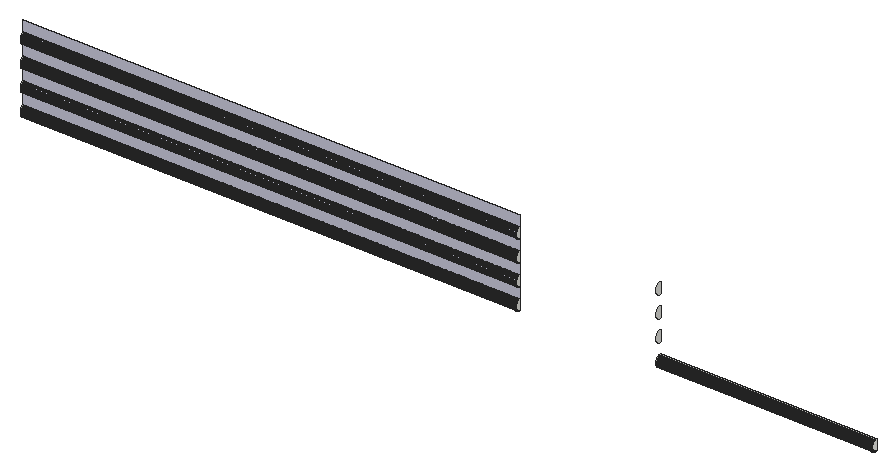
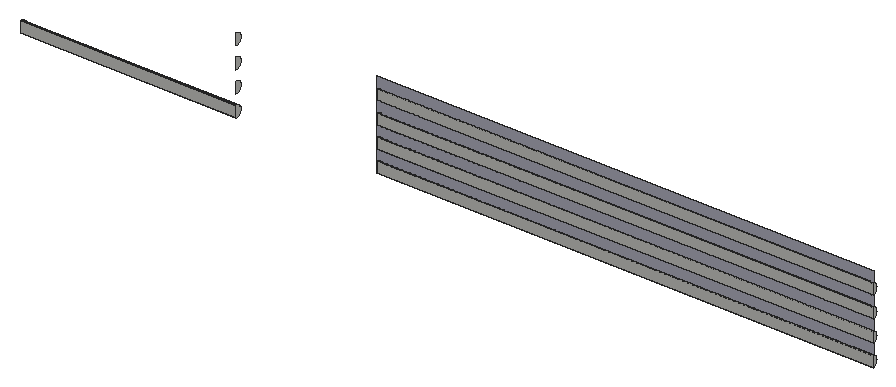
# SketchUp Ruby script. Lengths in millimetres.
U = 1.mm
M = Sketchup.active_model
def pt(a) = Geom::Point3d.new(a.map { |v| v * U })
def face(e, loops, mat)
  f = e.add_face(loops[0].map { |a| pt(a) })
  loops[1..].each { |l| e.add_face(l.map { |a| pt(a) }).erase! }
  f.material = f.back_material = mat if mat
  f
end
# faces: each face lists its corners as indices into pts; further lists are holes
def faces(e, pts, list, mat = nil) = list.each { |f| face(e, (f[0].is_a?(Array) ? f : [f]).map { |l| l.map { |i| pts[i] } }, mat) }
# xy, xz, yz: faces in a plane at the given z, y or x. An outline is a flat list of corners, or four numbers for a rectangle; further outlines are holes
def ring(l) = l.size == 4 ? [[l[0], l[1]], [l[2], l[1]], [l[2], l[3]], [l[0], l[3]]] : l.each_slice(2).to_a
def flat(e, list, mat, &to3) = list.each { |f| face(e, (f[0].is_a?(Array) ? f : [f]).map { |l| ring(l).map { |u, v| to3.(u, v) } }, mat) }
def xy(e, z, list, mat = nil) = flat(e, list, mat) { |x, y| [x, y, z] }
def xz(e, y, list, mat = nil) = flat(e, list, mat) { |x, z| [x, y, z] }
def yz(e, x, list, mat = nil) = flat(e, list, mat) { |y, z| [x, y, z] }
def lines(e, pts, list) = list.each { |a, b| e.add_line(pt(pts[a]), pt(pts[b])) }
# prism: a flat outline (further loops are holes) pulled along v
def prism(e, loops, v, mat = nil)
  f = face(e, loops, mat); d = Geom::Vector3d.new(v.map { |x| x * U })
  f.pushpull(f.normal.samedirection?(d) ? d.length : -d.length)
end
def box(e, o, s, mat = nil) = prism(e, [[o, [o[0] + s[0], o[1], o[2]], [o[0] + s[0], o[1] + s[1], o[2]], [o[0], o[1] + s[1], o[2]]]], [0, 0, s[2]], mat)
def at(x, y, z, deg = 0) = Geom::Transformation.translation(pt([x, y, z])) * Geom::Transformation.rotation(ORIGIN, Z_AXIS, deg.degrees)
def axes(o, x, y, z) = Geom::Transformation.new([*x, 0, *y, 0, *z, 0, *pt(o).to_a, 1])
def part(name) = M.definitions.add(name)
# library, detail: a bought-in or finely detailed component or shape, given as its bounding box
def library(name, o, s) = part(name).tap { |d| box(d.entities, o, s) }
def detail(e, o, s) = box(e.add_group.entities, o, s)
def put(e, d, t, mat = nil) = e.add_instance(d, t).tap { |i| i.material = mat if mat }
def group(e, t, mat = nil) = e.add_group.tap { |g| g.transformation = t; g.material = mat if mat }.entities
root = M.entities
M.materials.add("[0116_Lavender]").color = [197, 197, 214]
xz(root,16548.1,[[11038.5,8702.7,25059.3,9007.5],[29021.7,8702.7,35117.7,9007.5],[11038.5,9312.3,25059.3,9617.1],[11038.5,9921.9,25059.3,10226.7],[11038.5,10531.5,25059.3,10836.3]])
xz(root,16548.1,[[11038.5,9007.5,25059.3,9312.3],[11038.5,9617.1,25059.3,9921.9],[11038.5,10226.7,25059.3,10531.5],[11038.5,10836.3,25059.3,11141.1]],"[0116_Lavender]")
yz(root,11038.5,[[16548.1,8702.7,16536.2,8708,16524.8,8714.3,16514,8721.4,16503.7,8729.4,16494.1,8738.2,16485.2,8747.7,16477.1,8757.8,16469.8,8768.6,16463.4,8779.9,16458,8791.7,16453.4,8803.9,16449.9,8816.4,16447.3,8829.2,16445.8,8842.1,16445.3,8855.1,16445.8,8868.1,16447.3,8881,16449.9,8893.7,16453.4,8906.2,16458,8918.4,16463.4,8930.2,16469.8,8941.5,16477.1,8952.3,16485.2,8962.5,16494.1,8972,16503.7,8980.8,16514,8988.7,16524.8,8995.9,16536.2,9002.1,16548.1,9007.5],[16548.1,9312.3,16536.2,9317.6,16524.8,9323.9,16514,9331,16503.7,9339,16494.1,9347.8,16485.2,9357.3,16477.1,9367.4,16469.8,9378.2,16463.4,9389.5,16458,9401.3,16453.4,9413.5,16449.9,9426,16447.3,9438.8,16445.8,9451.7,16445.3,9464.7,16445.8,9477.7,16447.3,9490.6,16449.9,9503.3,16453.4,9515.8,16458,9528,16463.4,9539.8,16469.8,9551.1,16477.1,9561.9,16485.2,9572.1,16494.1,9581.6,16503.7,9590.4,16514,9598.3,16524.8,9605.5,16536.2,9611.7,16548.1,9617.1],[16548.1,9921.9,16536.2,9927.2,16524.8,9933.5,16514,9940.6,16503.7,9948.6,16494.1,9957.4,16485.2,9966.9,16477.1,9977,16469.8,9987.8,16463.4,9999.1,16458,10010.9,16453.4,10023.1,16449.9,10035.6,16447.3,10048.4,16445.8,10061.3,16445.3,10074.3,16445.8,10087.3,16447.3,10100.2,16449.9,10112.9,16453.4,10125.4,16458,10137.6,16463.4,10149.4,16469.8,10160.7,16477.1,10171.5,16485.2,10181.7,16494.1,10191.2,16503.7,10200,16514,10207.9,16524.8,10215.1,16536.2,10221.3,16548.1,10226.7],[16548.1,10531.5,16536.2,10536.8,16524.8,10543.1,16514,10550.2,16503.7,10558.2,16494.1,10567,16485.2,10576.5,16477.1,10586.6,16469.8,10597.4,16463.4,10608.7,16458,10620.5,16453.4,10632.7,16449.9,10645.2,16447.3,10658,16445.8,10670.9,16445.3,10683.9,16445.8,10696.9,16447.3,10709.8,16449.9,10722.5,16453.4,10735,16458,10747.2,16463.4,10759,16469.8,10770.3,16477.1,10781.1,16485.2,10791.3,16494.1,10800.8,16503.7,10809.6,16514,10817.5,16524.8,10824.7,16536.2,10830.9,16548.1,10836.3]])
yz(root,25059.3,[[16548.1,8702.7,16548.1,9007.5,16536.2,9002.1,16524.8,8995.9,16514,8988.7,16503.7,8980.8,16494.1,8972,16485.2,8962.5,16477.1,8952.3,16469.8,8941.5,16463.4,8930.2,16458,8918.4,16453.4,8906.2,16449.9,8893.7,16447.3,8881,16445.8,8868.1,16445.3,8855.1,16445.8,8842.1,16447.3,8829.2,16449.9,8816.4,16453.4,8803.9,16458,8791.7,16463.4,8779.9,16469.8,8768.6,16477.1,8757.8,16485.2,8747.7,16494.1,8738.2,16503.7,8729.4,16514,8721.4,16524.8,8714.3,16536.2,8708],[16548.1,9312.3,16548.1,9617.1,16536.2,9611.7,16524.8,9605.5,16514,9598.3,16503.7,9590.4,16494.1,9581.6,16485.2,9572.1,16477.1,9561.9,16469.8,9551.1,16463.4,9539.8,16458,9528,16453.4,9515.8,16449.9,9503.3,16447.3,9490.6,16445.8,9477.7,16445.3,9464.7,16445.8,9451.7,16447.3,9438.8,16449.9,9426,16453.4,9413.5,16458,9401.3,16463.4,9389.5,16469.8,9378.2,16477.1,9367.4,16485.2,9357.3,16494.1,9347.8,16503.7,9339,16514,9331,16524.8,9323.9,16536.2,9317.6],[16548.1,9921.9,16548.1,10226.7,16536.2,10221.3,16524.8,10215.1,16514,10207.9,16503.7,10200,16494.1,10191.2,16485.2,10181.7,16477.1,10171.5,16469.8,10160.7,16463.4,10149.4,16458,10137.6,16453.4,10125.4,16449.9,10112.9,16447.3,10100.2,16445.8,10087.3,16445.3,10074.3,16445.8,10061.3,16447.3,10048.4,16449.9,10035.6,16453.4,10023.1,16458,10010.9,16463.4,9999.1,16469.8,9987.8,16477.1,9977,16485.2,9966.9,16494.1,9957.4,16503.7,9948.6,16514,9940.6,16524.8,9933.5,16536.2,9927.2],[16548.1,10531.5,16548.1,10836.3,16536.2,10830.9,16524.8,10824.7,16514,10817.5,16503.7,10809.6,16494.1,10800.8,16485.2,10791.3,16477.1,10781.1,16469.8,10770.3,16463.4,10759,16458,10747.2,16453.4,10735,16449.9,10722.5,16447.3,10709.8,16445.8,10696.9,16445.3,10683.9,16445.8,10670.9,16447.3,10658,16449.9,10645.2,16453.4,10632.7,16458,10620.5,16463.4,10608.7,16469.8,10597.4,16477.1,10586.6,16485.2,10576.5,16494.1,10567,16503.7,10558.2,16514,10550.2,16524.8,10543.1,16536.2,10536.8]])
yz(root,29021.7,[[16548.1,8702.7,16540.1,8702.9,16532.2,8703.5,16524.3,8704.6,16516.4,8706,16508.7,8707.9,16501,8710.1,16493.5,8712.8,16486.1,8715.9,16478.9,8719.3,16471.9,8723.1,16465.1,8727.3,16458.5,8731.8,16452.2,8736.6,16446.1,8741.8,16440.3,8747.3,16434.8,8753.1,16429.7,8759.2,16424.8,8765.5,16420.3,8772.1,16416.1,8778.9,16412.3,8785.9,16408.9,8793.1,16405.8,8800.5,16403.2,8808,16400.9,8815.6,16399,8823.4,16397.6,8831.2,16396.5,8839.1,16395.9,8847.1,16395.7,8855.1,16395.9,8863.1,16396.5,8871,16397.6,8878.9,16399,8886.8,16400.9,8894.5,16403.2,8902.2,16405.8,8909.7,16408.9,8917.1,16412.3,8924.3,16416.1,8931.3,16420.3,8938.1,16424.8,8944.7,16429.7,8951,16434.8,8957.1,16440.3,8962.8,16446.1,8968.3,16452.2,8973.5,16458.5,8978.4,16465.1,8982.9,16471.9,8987.1,16478.9,8990.9,16486.1,8994.3,16493.5,8997.4,16501,9000,16508.7,9002.3,16516.4,9004.1,16524.3,9005.6,16532.2,9006.6,16540.1,9007.3,16548.1,9007.5],[16548.1,9312.3,16540.1,9312.5,16532.2,9313.1,16524.3,9314.2,16516.4,9315.6,16508.7,9317.5,16501,9319.7,16493.5,9322.4,16486.1,9325.5,16478.9,9328.9,16471.9,9332.7,16465.1,9336.9,16458.5,9341.4,16452.2,9346.2,16446.1,9351.4,16440.3,9356.9,16434.8,9362.7,16429.7,9368.8,16424.8,9375.1,16420.3,9381.7,16416.1,9388.5,16412.3,9395.5,16408.9,9402.7,16405.8,9410.1,16403.2,9417.6,16400.9,9425.2,16399,9433,16397.6,9440.8,16396.5,9448.7,16395.9,9456.7,16395.7,9464.7,16395.9,9472.7,16396.5,9480.6,16397.6,9488.5,16399,9496.4,16400.9,9504.1,16403.2,9511.8,16405.8,9519.3,16408.9,9526.7,16412.3,9533.9,16416.1,9540.9,16420.3,9547.7,16424.8,9554.3,16429.7,9560.6,16434.8,9566.7,16440.3,9572.4,16446.1,9577.9,16452.2,9583.1,16458.5,9588,16465.1,9592.5,16471.9,9596.7,16478.9,9600.5,16486.1,9603.9,16493.5,9607,16501,9609.6,16508.7,9611.9,16516.4,9613.7,16524.3,9615.2,16532.2,9616.2,16540.1,9616.9,16548.1,9617.1],[16548.1,9921.9,16540.1,9922.1,16532.2,9922.7,16524.3,9923.8,16516.4,9925.2,16508.7,9927.1,16501,9929.3,16493.5,9932,16486.1,9935.1,16478.9,9938.5,16471.9,9942.3,16465.1,9946.5,16458.5,9951,16452.2,9955.8,16446.1,9961,16440.3,9966.5,16434.8,9972.3,16429.7,9978.4,16424.8,9984.7,16420.3,9991.3,16416.1,9998.1,16412.3,10005.1,16408.9,10012.3,16405.8,10019.7,16403.2,10027.2,16400.9,10034.8,16399,10042.6,16397.6,10050.4,16396.5,10058.3,16395.9,10066.3,16395.7,10074.3,16395.9,10082.3,16396.5,10090.2,16397.6,10098.1,16399,10106,16400.9,10113.7,16403.2,10121.4,16405.8,10128.9,16408.9,10136.3,16412.3,10143.5,16416.1,10150.5,16420.3,10157.3,16424.8,10163.9,16429.7,10170.2,16434.8,10176.3,16440.3,10182,16446.1,10187.5,16452.2,10192.7,16458.5,10197.6,16465.1,10202.1,16471.9,10206.3,16478.9,10210.1,16486.1,10213.5,16493.5,10216.6,16501,10219.2,16508.7,10221.5,16516.4,10223.3,16524.3,10224.8,16532.2,10225.8,16540.1,10226.5,16548.1,10226.7],[16548.1,10531.5,16540.1,10531.7,16532.2,10532.3,16524.3,10533.4,16516.4,10534.8,16508.7,10536.7,16501,10538.9,16493.5,10541.6,16486.1,10544.7,16478.9,10548.1,16471.9,10551.9,16465.1,10556.1,16458.5,10560.6,16452.2,10565.4,16446.1,10570.6,16440.3,10576.1,16434.8,10581.9,16429.7,10588,16424.8,10594.3,16420.3,10600.9,16416.1,10607.7,16412.3,10614.7,16408.9,10621.9,16405.8,10629.3,16403.2,10636.8,16400.9,10644.4,16399,10652.2,16397.6,10660,16396.5,10667.9,16395.9,10675.9,16395.7,10683.9,16395.9,10691.9,16396.5,10699.8,16397.6,10707.7,16399,10715.6,16400.9,10723.3,16403.2,10731,16405.8,10738.5,16408.9,10745.9,16412.3,10753.1,16416.1,10760.1,16420.3,10766.9,16424.8,10773.5,16429.7,10779.8,16434.8,10785.9,16440.3,10791.6,16446.1,10797.1,16452.2,10802.3,16458.5,10807.2,16465.1,10811.7,16471.9,10815.9,16478.9,10819.7,16486.1,10823.1,16493.5,10826.2,16501,10828.8,16508.7,10831.1,16516.4,10832.9,16524.3,10834.4,16532.2,10835.4,16540.1,10836.1,16548.1,10836.3]])
p = [[25059.3,16548.1,8702.7],[25059.3,16536.2,8708],[11038.5,16536.2,8708],[11038.5,16548.1,8702.7],[35117.7,16548.1,8702.7],[35117.7,16540.1,8702.9],
  [29021.7,16540.1,8702.9],[29021.7,16548.1,8702.7],[35117.7,16532.2,8703.5],[29021.7,16532.2,8703.5],[35117.7,16524.3,8704.6],[29021.7,16524.3,8704.6],
  [35117.7,16516.4,8706],[29021.7,16516.4,8706],[35117.7,16508.7,8707.9],[29021.7,16508.7,8707.9],[35117.7,16501,8710.1],[29021.7,16501,8710.1],
  [25059.3,16524.8,8714.3],[11038.5,16524.8,8714.3],[35117.7,16493.5,8712.8],[29021.7,16493.5,8712.8],[35117.7,16486.1,8715.9],[29021.7,16486.1,8715.9],
  [25059.3,16514,8721.4],[11038.5,16514,8721.4],[35117.7,16478.9,8719.3],[29021.7,16478.9,8719.3],[35117.7,16471.9,8723.1],[29021.7,16471.9,8723.1],
  [25059.3,16503.7,8729.4],[11038.5,16503.7,8729.4],[35117.7,16465.1,8727.3],[29021.7,16465.1,8727.3],[35117.7,16458.5,8731.8],[29021.7,16458.5,8731.8],
  [25059.3,16494.1,8738.2],[11038.5,16494.1,8738.2],[35117.7,16452.2,8736.6],[29021.7,16452.2,8736.6],[35117.7,16446.1,8741.8],[29021.7,16446.1,8741.8],
  [25059.3,16485.2,8747.7],[11038.5,16485.2,8747.7],[35117.7,16440.3,8747.3],[29021.7,16440.3,8747.3],[35117.7,16434.8,8753.1],[29021.7,16434.8,8753.1],
  [25059.3,16477.1,8757.8],[11038.5,16477.1,8757.8],[35117.7,16429.7,8759.2],[29021.7,16429.7,8759.2],[25059.3,16469.8,8768.6],[11038.5,16469.8,8768.6],
  [35117.7,16424.8,8765.5],[29021.7,16424.8,8765.5],[35117.7,16420.3,8772.1],[29021.7,16420.3,8772.1],[25059.3,16463.4,8779.9],[11038.5,16463.4,8779.9],
  [35117.7,16416.1,8778.9],[29021.7,16416.1,8778.9],[35117.7,16412.3,8785.9],[29021.7,16412.3,8785.9],[25059.3,16458,8791.7],[11038.5,16458,8791.7],
  [35117.7,16408.9,8793.1],[29021.7,16408.9,8793.1],[25059.3,16453.4,8803.9],[11038.5,16453.4,8803.9],[35117.7,16405.8,8800.5],[29021.7,16405.8,8800.5],
  [35117.7,16403.2,8808],[29021.7,16403.2,8808],[25059.3,16449.9,8816.4],[11038.5,16449.9,8816.4],[35117.7,16400.9,8815.6],[29021.7,16400.9,8815.6],
  [35117.7,16399,8823.4],[29021.7,16399,8823.4],[25059.3,16447.3,8829.2],[11038.5,16447.3,8829.2],[35117.7,16397.6,8831.2],[29021.7,16397.6,8831.2],
  [25059.3,16445.8,8842.1],[11038.5,16445.8,8842.1],[35117.7,16396.5,8839.1],[29021.7,16396.5,8839.1],[35117.7,16395.9,8847.1],[29021.7,16395.9,8847.1],
  [25059.3,16445.3,8855.1],[11038.5,16445.3,8855.1],[35117.7,16395.7,8855.1],[29021.7,16395.7,8855.1],[35117.7,16395.9,8863.1],[29021.7,16395.9,8863.1],
  [25059.3,16445.8,8868.1],[11038.5,16445.8,8868.1],[35117.7,16396.5,8871],[29021.7,16396.5,8871],[25059.3,16447.3,8881],[11038.5,16447.3,8881],
  [35117.7,16397.6,8878.9],[29021.7,16397.6,8878.9],[35117.7,16399,8886.8],[29021.7,16399,8886.8],[25059.3,16449.9,8893.7],[11038.5,16449.9,8893.7],
  [35117.7,16400.9,8894.5],[29021.7,16400.9,8894.5],[25059.3,16453.4,8906.2],[11038.5,16453.4,8906.2],[35117.7,16403.2,8902.2],[29021.7,16403.2,8902.2],
  [35117.7,16405.8,8909.7],[29021.7,16405.8,8909.7],[25059.3,16458,8918.4],[11038.5,16458,8918.4],[35117.7,16408.9,8917.1],[29021.7,16408.9,8917.1],
  [35117.7,16412.3,8924.3],[29021.7,16412.3,8924.3],[25059.3,16463.4,8930.2],[11038.5,16463.4,8930.2],[35117.7,16416.1,8931.3],[29021.7,16416.1,8931.3],
  [25059.3,16469.8,8941.5],[11038.5,16469.8,8941.5],[35117.7,16420.3,8938.1],[29021.7,16420.3,8938.1],[35117.7,16424.8,8944.7],[29021.7,16424.8,8944.7],
  [25059.3,16477.1,8952.3],[11038.5,16477.1,8952.3],[35117.7,16429.7,8951],[29021.7,16429.7,8951],[35117.7,16434.8,8957.1],[29021.7,16434.8,8957.1],
  [25059.3,16485.2,8962.5],[11038.5,16485.2,8962.5],[35117.7,16440.3,8962.8],[29021.7,16440.3,8962.8],[25059.3,16494.1,8972],[11038.5,16494.1,8972],
  [35117.7,16446.1,8968.3],[29021.7,16446.1,8968.3],[35117.7,16452.2,8973.5],[29021.7,16452.2,8973.5],[25059.3,16503.7,8980.8],[11038.5,16503.7,8980.8],
  [35117.7,16458.5,8978.4],[29021.7,16458.5,8978.4],[35117.7,16465.1,8982.9],[29021.7,16465.1,8982.9],[25059.3,16514,8988.7],[11038.5,16514,8988.7],
  [35117.7,16471.9,8987.1],[29021.7,16471.9,8987.1],[35117.7,16478.9,8990.9],[29021.7,16478.9,8990.9],[25059.3,16524.8,8995.9],[11038.5,16524.8,8995.9],
  [35117.7,16486.1,8994.3],[29021.7,16486.1,8994.3],[35117.7,16493.5,8997.4],[29021.7,16493.5,8997.4],[25059.3,16536.2,9002.1],[11038.5,16536.2,9002.1],
  [35117.7,16501,9000],[29021.7,16501,9000],[35117.7,16508.7,9002.3],[29021.7,16508.7,9002.3],[25059.3,16548.1,9007.5],[11038.5,16548.1,9007.5],
  [25059.3,16548.1,9312.3],[25059.3,16536.2,9317.6],[11038.5,16536.2,9317.6],[11038.5,16548.1,9312.3],[25059.3,16524.8,9323.9],[11038.5,16524.8,9323.9],
  [25059.3,16514,9331],[11038.5,16514,9331],[25059.3,16503.7,9339],[11038.5,16503.7,9339],[25059.3,16494.1,9347.8],[11038.5,16494.1,9347.8],
  [25059.3,16485.2,9357.3],[11038.5,16485.2,9357.3],[25059.3,16477.1,9367.4],[11038.5,16477.1,9367.4],[25059.3,16469.8,9378.2],[11038.5,16469.8,9378.2],
  [25059.3,16463.4,9389.5],[11038.5,16463.4,9389.5],[25059.3,16458,9401.3],[11038.5,16458,9401.3],[25059.3,16453.4,9413.5],[11038.5,16453.4,9413.5],
  [25059.3,16449.9,9426],[11038.5,16449.9,9426],[25059.3,16447.3,9438.8],[11038.5,16447.3,9438.8],[25059.3,16445.8,9451.7],[11038.5,16445.8,9451.7],
  [25059.3,16445.3,9464.7],[11038.5,16445.3,9464.7],[25059.3,16445.8,9477.7],[11038.5,16445.8,9477.7],[25059.3,16447.3,9490.6],[11038.5,16447.3,9490.6],
  [25059.3,16449.9,9503.3],[11038.5,16449.9,9503.3],[25059.3,16453.4,9515.8],[11038.5,16453.4,9515.8],[25059.3,16458,9528],[11038.5,16458,9528],
  [25059.3,16463.4,9539.8],[11038.5,16463.4,9539.8],[25059.3,16469.8,9551.1],[11038.5,16469.8,9551.1],[25059.3,16477.1,9561.9],[11038.5,16477.1,9561.9],
  [25059.3,16485.2,9572.1],[11038.5,16485.2,9572.1],[25059.3,16494.1,9581.6],[11038.5,16494.1,9581.6],[25059.3,16503.7,9590.4],[11038.5,16503.7,9590.4],
  [25059.3,16514,9598.3],[11038.5,16514,9598.3],[25059.3,16524.8,9605.5],[11038.5,16524.8,9605.5],[25059.3,16536.2,9611.7],[11038.5,16536.2,9611.7],
  [25059.3,16548.1,9617.1],[11038.5,16548.1,9617.1],[25059.3,16548.1,9921.9],[25059.3,16536.2,9927.2],[11038.5,16536.2,9927.2],[11038.5,16548.1,9921.9],
  [25059.3,16524.8,9933.5],[11038.5,16524.8,9933.5],[25059.3,16514,9940.6],[11038.5,16514,9940.6],[25059.3,16503.7,9948.6],[11038.5,16503.7,9948.6],
  [25059.3,16494.1,9957.4],[11038.5,16494.1,9957.4],[25059.3,16485.2,9966.9],[11038.5,16485.2,9966.9],[25059.3,16477.1,9977],[11038.5,16477.1,9977],
  [25059.3,16469.8,9987.8],[11038.5,16469.8,9987.8],[25059.3,16463.4,9999.1],[11038.5,16463.4,9999.1],[25059.3,16458,10010.9],[11038.5,16458,10010.9],
  [25059.3,16453.4,10023.1],[11038.5,16453.4,10023.1],[25059.3,16449.9,10035.6],[11038.5,16449.9,10035.6],[25059.3,16447.3,10048.4],[11038.5,16447.3,10048.4],
  [25059.3,16445.8,10061.3],[11038.5,16445.8,10061.3],[25059.3,16445.3,10074.3],[11038.5,16445.3,10074.3],[25059.3,16445.8,10087.3],[11038.5,16445.8,10087.3],
  [25059.3,16447.3,10100.2],[11038.5,16447.3,10100.2],[25059.3,16449.9,10112.9],[11038.5,16449.9,10112.9],[25059.3,16453.4,10125.4],[11038.5,16453.4,10125.4],
  [25059.3,16458,10137.6],[11038.5,16458,10137.6],[25059.3,16463.4,10149.4],[11038.5,16463.4,10149.4],[25059.3,16469.8,10160.7],[11038.5,16469.8,10160.7],
  [25059.3,16477.1,10171.5],[11038.5,16477.1,10171.5],[25059.3,16485.2,10181.7],[11038.5,16485.2,10181.7],[25059.3,16494.1,10191.2],[11038.5,16494.1,10191.2],
  [25059.3,16503.7,10200],[11038.5,16503.7,10200],[25059.3,16514,10207.9],[11038.5,16514,10207.9],[25059.3,16524.8,10215.1],[11038.5,16524.8,10215.1],
  [25059.3,16536.2,10221.3],[11038.5,16536.2,10221.3],[25059.3,16548.1,10226.7],[11038.5,16548.1,10226.7],[25059.3,16548.1,10531.5],[25059.3,16536.2,10536.8],
  [11038.5,16536.2,10536.8],[11038.5,16548.1,10531.5],[25059.3,16524.8,10543.1],[11038.5,16524.8,10543.1],[25059.3,16514,10550.2],[11038.5,16514,10550.2],
  [25059.3,16503.7,10558.2],[11038.5,16503.7,10558.2],[25059.3,16494.1,10567],[11038.5,16494.1,10567],[25059.3,16485.2,10576.5],[11038.5,16485.2,10576.5],
  [25059.3,16477.1,10586.6],[11038.5,16477.1,10586.6],[25059.3,16469.8,10597.4],[11038.5,16469.8,10597.4],[25059.3,16463.4,10608.7],[11038.5,16463.4,10608.7],
  [25059.3,16458,10620.5],[11038.5,16458,10620.5],[25059.3,16453.4,10632.7],[11038.5,16453.4,10632.7],[25059.3,16449.9,10645.2],[11038.5,16449.9,10645.2],
  [25059.3,16447.3,10658],[11038.5,16447.3,10658],[25059.3,16445.8,10670.9],[11038.5,16445.8,10670.9],[25059.3,16445.3,10683.9],[11038.5,16445.3,10683.9],
  [25059.3,16445.8,10696.9],[11038.5,16445.8,10696.9],[25059.3,16447.3,10709.8],[11038.5,16447.3,10709.8],[25059.3,16449.9,10722.5],[11038.5,16449.9,10722.5],
  [25059.3,16453.4,10735],[11038.5,16453.4,10735],[25059.3,16458,10747.2],[11038.5,16458,10747.2],[25059.3,16463.4,10759],[11038.5,16463.4,10759],
  [25059.3,16469.8,10770.3],[11038.5,16469.8,10770.3],[25059.3,16477.1,10781.1],[11038.5,16477.1,10781.1],[25059.3,16485.2,10791.3],[11038.5,16485.2,10791.3],
  [25059.3,16494.1,10800.8],[11038.5,16494.1,10800.8],[25059.3,16503.7,10809.6],[11038.5,16503.7,10809.6],[25059.3,16514,10817.5],[11038.5,16514,10817.5],
  [25059.3,16524.8,10824.7],[11038.5,16524.8,10824.7],[25059.3,16536.2,10830.9],[11038.5,16536.2,10830.9],[25059.3,16548.1,10836.3],[11038.5,16548.1,10836.3]]
faces(root,p,[[0,1,2,3],[4,5,6,7],[5,8,9,6],[8,10,11,9],[10,12,13,11],[12,14,15,13],[14,16,17,15],[1,18,19,2],
  [16,20,21,17],[20,22,23,21],[18,24,25,19],[22,26,27,23],[26,28,29,27],[24,30,31,25],[28,32,33,29],[32,34,35,33],
  [30,36,37,31],[34,38,39,35],[38,40,41,39],[36,42,43,37],[40,44,45,41],[44,46,47,45],[42,48,49,43],[46,50,51,47],
  [48,52,53,49],[50,54,55,51],[54,56,57,55],[52,58,59,53],[56,60,61,57],[60,62,63,61],[58,64,65,59],[62,66,67,63],
  [64,68,69,65],[66,70,71,67],[70,72,73,71],[68,74,75,69],[72,76,77,73],[76,78,79,77],[74,80,81,75],[78,82,83,79],
  [80,84,85,81],[82,86,87,83],[86,88,89,87],[84,90,91,85],[88,92,93,89],[92,94,95,93],[90,96,97,91],[94,98,99,95],
  [96,100,101,97],[98,102,103,99],[102,104,105,103],[100,106,107,101],[104,108,109,105],[106,110,111,107],[108,112,113,109],[112,114,115,113],
  [110,116,117,111],[114,118,119,115],[118,120,121,119],[116,122,123,117],[120,124,125,121],[122,126,127,123],[124,128,129,125],[128,130,131,129],
  [126,132,133,127],[130,134,135,131],[134,136,137,135],[132,138,139,133],[136,140,141,137],[138,142,143,139],[140,144,145,141],[144,146,147,145],
  [142,148,149,143],[146,150,151,147],[150,152,153,151],[148,154,155,149],[152,156,157,153],[156,158,159,157],[154,160,161,155],[158,162,163,159],
  [162,164,165,163],[160,166,167,161],[164,168,169,165],[168,170,171,169],[166,172,173,167],[174,175,176,177],[175,178,179,176],[178,180,181,179],
  [180,182,183,181],[182,184,185,183],[184,186,187,185],[186,188,189,187],[188,190,191,189],[190,192,193,191],[192,194,195,193],[194,196,197,195],
  [196,198,199,197],[198,200,201,199],[200,202,203,201],[202,204,205,203],[204,206,207,205],[206,208,209,207],[208,210,211,209],[210,212,213,211],
  [212,214,215,213],[214,216,217,215],[216,218,219,217],[218,220,221,219],[220,222,223,221],[222,224,225,223],[224,226,227,225],[226,228,229,227],
  [228,230,231,229],[230,232,233,231],[232,234,235,233],[236,237,238,239],[237,240,241,238],[240,242,243,241],[242,244,245,243],[244,246,247,245],
  [246,248,249,247],[248,250,251,249],[250,252,253,251],[252,254,255,253],[254,256,257,255],[256,258,259,257],[258,260,261,259],[260,262,263,261],
  [262,264,265,263],[264,266,267,265],[266,268,269,267],[268,270,271,269],[270,272,273,271],[272,274,275,273],[274,276,277,275],[276,278,279,277],
  [278,280,281,279],[280,282,283,281],[282,284,285,283],[284,286,287,285],[286,288,289,287],[288,290,291,289],[290,292,293,291],[292,294,295,293],
  [294,296,297,295],[298,299,300,301],[299,302,303,300],[302,304,305,303],[304,306,307,305],[306,308,309,307],[308,310,311,309],[310,312,313,311],
  [312,314,315,313],[314,316,317,315],[316,318,319,317],[318,320,321,319],[320,322,323,321],[322,324,325,323],[324,326,327,325],[326,328,329,327],
  [328,330,331,329],[330,332,333,331],[332,334,335,333],[334,336,337,335],[336,338,339,337],[338,340,341,339],[340,342,343,341],[342,344,345,343],
  [344,346,347,345],[346,348,349,347],[348,350,351,349],[350,352,353,351],[352,354,355,353],[354,356,357,355],[356,358,359,357]],"[0116_Lavender]")
